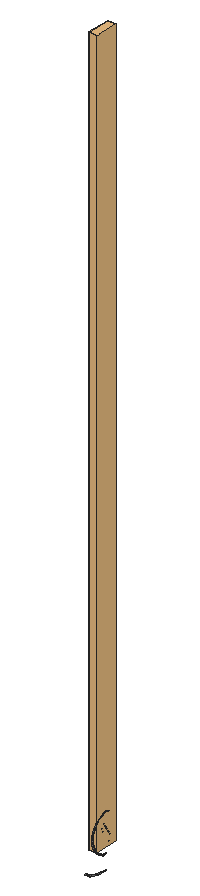
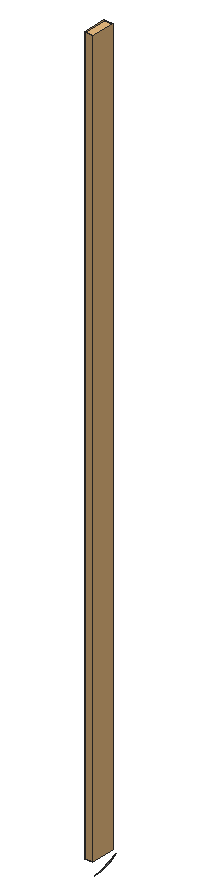
# SketchUp Ruby script. Lengths in inches.
U = 1.inch
M = Sketchup.active_model
def pt(a) = Geom::Point3d.new(a.map { |v| v * U })
def face(e, loops, mat)
  f = e.add_face(loops[0].map { |a| pt(a) })
  loops[1..].each { |l| e.add_face(l.map { |a| pt(a) }).erase! }
  f.material = f.back_material = mat if mat
  f
end
# faces: each face lists its corners as indices into pts; further lists are holes
def faces(e, pts, list, mat = nil) = list.each { |f| face(e, (f[0].is_a?(Array) ? f : [f]).map { |l| l.map { |i| pts[i] } }, mat) }
# xy, xz, yz: faces in a plane at the given z, y or x. An outline is a flat list of corners, or four numbers for a rectangle; further outlines are holes
def ring(l) = l.size == 4 ? [[l[0], l[1]], [l[2], l[1]], [l[2], l[3]], [l[0], l[3]]] : l.each_slice(2).to_a
def flat(e, list, mat, &to3) = list.each { |f| face(e, (f[0].is_a?(Array) ? f : [f]).map { |l| ring(l).map { |u, v| to3.(u, v) } }, mat) }
def xy(e, z, list, mat = nil) = flat(e, list, mat) { |x, y| [x, y, z] }
def xz(e, y, list, mat = nil) = flat(e, list, mat) { |x, z| [x, y, z] }
def yz(e, x, list, mat = nil) = flat(e, list, mat) { |y, z| [x, y, z] }
def lines(e, pts, list) = list.each { |a, b| e.add_line(pt(pts[a]), pt(pts[b])) }
# prism: a flat outline (further loops are holes) pulled along v
def prism(e, loops, v, mat = nil)
  f = face(e, loops, mat); d = Geom::Vector3d.new(v.map { |x| x * U })
  f.pushpull(f.normal.samedirection?(d) ? d.length : -d.length)
end
def box(e, o, s, mat = nil) = prism(e, [[o, [o[0] + s[0], o[1], o[2]], [o[0] + s[0], o[1] + s[1], o[2]], [o[0], o[1] + s[1], o[2]]]], [0, 0, s[2]], mat)
def at(x, y, z, deg = 0) = Geom::Transformation.translation(pt([x, y, z])) * Geom::Transformation.rotation(ORIGIN, Z_AXIS, deg.degrees)
def axes(o, x, y, z) = Geom::Transformation.new([*x, 0, *y, 0, *z, 0, *pt(o).to_a, 1])
def part(name) = M.definitions.add(name)
# library, detail: a bought-in or finely detailed component or shape, given as its bounding box
def library(name, o, s) = part(name).tap { |d| box(d.entities, o, s) }
def detail(e, o, s) = box(e.add_group.entities, o, s)
def put(e, d, t, mat = nil) = e.add_instance(d, t).tap { |i| i.material = mat if mat }
def group(e, t, mat = nil) = e.add_group.tap { |g| g.transformation = t; g.material = mat if mat }.entities
root = M.entities
M.materials.add("Material \#1").color = [140, 140, 140]
c1 = part("3DGeom~5_Defintion")
xy(c1.entities,-225.24,[[-0.79,-499.98,-2.33,-499.64,7.45,-496.14],[-0.79,-499.98,7.45,-496.14,1.58,-499.88],[1.58,-499.88,7.45,-496.14,3.84,-499.16],[-2.33,-499.64,7.4,-485.75,7.45,-496.14],[3.84,-499.16,7.45,-496.14,5.85,-497.89],
  [7.45,-496.14,7.4,-485.75,8.24,-487.08],[7.45,-496.14,8.24,-487.08,8.96,-489.34],[7.45,-496.14,8.96,-489.34,9.0625,-491.71],[7.45,-496.14,9.0625,-491.71,8.55,-494.03],[-7.4,-496.08,-8.24,-494.76,2.32,-482.2],
  [-8.24,-494.76,-8.96,-492.5,2.32,-482.2],[-8.96,-492.5,-9.0625,-490.125,2.32,-482.2],[-9.0625,-490.125,-8.55,-487.81,2.32,-482.2],[-8.55,-487.81,-7.45,-485.7,2.32,-482.2],[-7.45,-485.7,-5.85,-483.95,2.32,-482.2],
  [-5.85,-483.95,-3.84,-482.68,2.32,-482.2],[-3.84,-482.68,-1.58,-481.96,2.32,-482.2],[2.32,-482.2,-1.58,-481.96,0.79,-481.86],[0,481.82,-2.35,482.13,-6.92,496.71],[0,481.82,-6.92,496.71,1.55,482.04],
  [-2.35,482.13,-4.55,483.04,-6.92,496.71],[-4.55,483.04,-6.43,484.49,-6.92,496.71],[-6.43,484.49,-7.88,486.37,-6.92,496.71],[6.92,485.12,-1.55,499.8125,7.88,495.47],[6.92,485.12,7.88,495.47,7.88,486.37],
  [-7.88,486.37,-8.79,488.57,-6.92,496.71],[7.88,486.37,7.88,495.47,8.79,488.57],[-8.79,488.57,-9.1,490.92,-6.92,496.71],[8.79,488.57,7.88,495.47,9.1,490.92],[-9.1,490.92,-8.79,493.28,-6.92,496.71],
  [9.1,490.92,7.88,495.47,8.79,493.28],[-8.79,493.28,-7.88,495.47,-6.92,496.71],[7.88,495.47,-1.55,499.8125,0,500.02],[7.88,495.47,0,500.02,2.35,499.71],[7.88,495.47,2.35,499.71,4.55,498.8],
  [7.88,495.47,4.55,498.8,6.43,497.35]],"Material \#1")
xy(c1.entities,-221.57,[[-2.33,-499.64,-5.22,-498.37,7.4,-485.75],[-5.22,-498.37,-7.4,-496.08,5.22,-483.47],[-5.22,-498.37,5.22,-483.47,7.4,-485.75],[-7.4,-496.08,2.32,-482.2,5.22,-483.47],[1.55,482.04,-6.92,496.71,-4.55,498.8],
  [1.55,482.04,-4.55,498.8,4.55,483.04],[4.55,483.04,-4.55,498.8,-1.55,499.8125],[4.55,483.04,-1.55,499.8125,6.92,485.12]],"Material \#1")
xy(c1.entities,38.05,[[-2.33,-499.64,7.4,-485.75,-5.22,-498.37],[-5.22,-498.37,5.22,-483.47,-7.4,-496.08],[-5.22,-498.37,7.4,-485.75,5.22,-483.47],[-7.4,-496.08,5.22,-483.47,2.32,-482.2],[1.55,482.04,-4.55,498.8,-6.92,496.71],
  [1.55,482.04,4.55,483.04,-4.55,498.8],[4.55,483.04,-1.55,499.8125,-4.55,498.8],[4.55,483.04,6.92,485.12,-1.55,499.8125]],"Material \#1")
xy(c1.entities,41.72,[[-0.79,-499.98,7.45,-496.14,-2.33,-499.64],[-0.79,-499.98,1.58,-499.88,7.45,-496.14],[1.58,-499.88,3.84,-499.16,7.45,-496.14],[-2.33,-499.64,7.45,-496.14,7.4,-485.75],[3.84,-499.16,5.85,-497.89,7.45,-496.14],
  [7.45,-496.14,8.24,-487.08,7.4,-485.75],[7.45,-496.14,8.55,-494.03,9.0625,-491.71],[7.45,-496.14,8.96,-489.34,8.24,-487.08],[7.45,-496.14,9.0625,-491.71,8.96,-489.34],[-7.4,-496.08,2.32,-482.2,-8.24,-494.76],
  [-8.24,-494.76,2.32,-482.2,-8.96,-492.5],[-8.96,-492.5,2.32,-482.2,-9.0625,-490.125],[-9.0625,-490.125,2.32,-482.2,-8.55,-487.81],[-8.55,-487.81,2.32,-482.2,-7.45,-485.7],[-7.45,-485.7,2.32,-482.2,-5.85,-483.95],
  [-5.85,-483.95,2.32,-482.2,-3.84,-482.68],[-3.84,-482.68,2.32,-482.2,-1.58,-481.96],[2.32,-482.2,0.79,-481.86,-1.58,-481.96],[0,481.82,-6.92,496.71,-2.35,482.13],[0,481.82,1.55,482.04,-6.92,496.71],
  [-2.35,482.13,-6.92,496.71,-4.55,483.04],[-4.55,483.04,-6.92,496.71,-6.43,484.49],[-6.43,484.49,-6.92,496.71,-7.88,486.37],[6.92,485.12,7.88,495.47,-1.55,499.8125],[6.92,485.12,7.88,486.37,7.88,495.47],
  [-7.88,486.37,-6.92,496.71,-8.79,488.57],[7.88,486.37,8.79,488.57,7.88,495.47],[-8.79,488.57,-6.92,496.71,-9.1,490.92],[8.79,488.57,9.1,490.92,7.88,495.47],[-9.1,490.92,-6.92,496.71,-8.79,493.28],
  [9.1,490.92,8.79,493.28,7.88,495.47],[-8.79,493.28,-6.92,496.71,-7.88,495.47],[7.88,495.47,0,500.02,-1.55,499.8125],[7.88,495.47,2.35,499.71,0,500.02],[7.88,495.47,4.55,498.8,2.35,499.71],
  [7.88,495.47,6.43,497.35,4.55,498.8]],"Material \#1")
c2 = library("3DGeom~4_Defintion",[-18.02,-499.97,-221.16],[36.04,1000,262.12])
yz(root,362.685,[[201.798,43.518,201.655,43.532,201.658,43.547],[201.798,43.518,201.658,43.547,201.798,43.533],[201.655,43.532,201.522,43.572,201.526,43.586],[201.655,43.532,201.526,43.586,201.658,43.547],[201.522,43.572,201.399,43.636,201.405,43.649],
  [201.522,43.572,201.405,43.649,201.526,43.586],[201.798,43.749,201.751,43.754,201.753,43.768],[201.798,43.749,201.753,43.768,201.798,43.764],[201.751,43.754,201.706,43.767,201.711,43.781],[201.751,43.754,201.711,43.781,201.753,43.768],
  [201.706,43.767,201.665,43.788,201.672,43.801],[201.706,43.767,201.672,43.801,201.711,43.781],[201.665,43.788,201.628,43.817,201.637,43.828],[201.665,43.788,201.637,43.828,201.672,43.801],[201.628,43.817,201.597,43.851,201.607,43.861],
  [201.628,43.817,201.607,43.861,201.637,43.828],[201.597,43.851,201.571,43.891,201.583,43.898],[201.597,43.851,201.583,43.898,201.607,43.861],[201.571,43.891,201.551,43.936,201.564,43.941],[201.571,43.891,201.564,43.941,201.583,43.898],
  [201.551,43.936,201.539,43.984,201.552,43.987],[201.551,43.936,201.552,43.987,201.564,43.941],[201.539,43.984,201.535,44.036,201.548,44.036],[201.539,43.984,201.548,44.036,201.552,43.987],[201.535,44.036,201.539,44.087,201.552,44.084],
  [201.535,44.036,201.552,44.084,201.548,44.036],[201.552,44.084,201.539,44.087,201.564,44.13],[201.539,44.087,201.551,44.135,201.564,44.13],[201.564,44.13,201.551,44.135,201.583,44.173],[201.551,44.135,201.571,44.18,201.583,44.173],
  [201.583,44.173,201.571,44.18,201.607,44.211],[201.571,44.18,201.597,44.22,201.607,44.211],[201.607,44.211,201.597,44.22,201.637,44.243],[201.597,44.22,201.628,44.255,201.637,44.243],[201.637,44.243,201.628,44.255,201.672,44.27],
  [201.628,44.255,201.665,44.283,201.672,44.27],[201.672,44.27,201.665,44.283,201.711,44.29],[201.665,44.283,201.706,44.304,201.711,44.29],[201.711,44.29,201.706,44.304,201.753,44.303],[201.753,44.303,201.706,44.304,201.751,44.318],
  [201.753,44.303,201.751,44.318,201.798,44.307],[201.842,44.303,201.798,44.307,201.798,44.322],[201.798,44.307,201.751,44.318,201.798,44.322]],"Material \#1")
p = [[362.566,201.821,43.942],[362.567,201.821,43.942],[362.567,201.725,44.091],[362.566,201.725,44.091],[362.685,201.821,43.942],[362.685,201.725,44.091],
  [362.684,201.725,44.091],[362.684,201.821,43.942],[362.566,201.858,43.883],[362.568,201.858,43.883],[362.568,201.838,43.914],[362.566,201.838,43.914],
  [362.685,201.858,43.883],[362.685,201.838,43.914],[362.684,201.838,43.914],[362.683,201.858,43.883],[362.566,201.889,43.953],[362.568,201.889,43.953],
  [362.568,201.908,43.922],[362.566,201.908,43.922],[362.568,201.886,43.899],[362.566,201.886,43.899],[362.685,201.889,43.953],[362.685,201.908,43.922],
  [362.683,201.908,43.922],[362.684,201.889,43.953],[362.685,201.886,43.899],[362.683,201.886,43.899],[362.566,201.775,44.129],[362.567,201.775,44.129],
  [362.567,201.871,43.98],[362.566,201.871,43.98],[362.685,201.775,44.129],[362.685,201.871,43.98],[362.684,201.871,43.98],[362.684,201.775,44.129],
  [362.568,201.707,44.119],[362.566,201.707,44.119],[362.568,201.687,44.149],[362.566,201.687,44.149],[362.568,201.71,44.172],[362.566,201.71,44.172],
  [362.685,201.707,44.119],[362.684,201.707,44.119],[362.685,201.687,44.149],[362.683,201.687,44.149],[362.685,201.71,44.172],[362.683,201.71,44.172],
  [362.566,201.757,44.157],[362.568,201.757,44.157],[362.685,201.757,44.157],[362.684,201.757,44.157],[362.568,201.737,44.188],[362.566,201.737,44.188],
  [362.685,201.737,44.188],[362.683,201.737,44.188]]
faces(root,p,[[0,1,2],[2,3,0],[4,5,6],[6,7,4],[8,9,10],[10,11,8],[11,10,1],[1,0,11],
  [12,13,14],[14,15,12],[13,4,7],[7,14,13],[16,17,18],[18,19,16],[19,18,20],[20,21,19],
  [21,20,9],[9,8,21],[22,23,24],[24,25,22],[23,26,27],[27,24,23],[26,12,15],[15,27,26],
  [28,29,30],[30,31,28],[32,33,34],[34,35,32],[31,30,17],[17,16,31],[33,22,25],[25,34,33],
  [3,2,36],[36,37,3],[37,36,38],[38,39,37],[39,38,40],[40,41,39],[5,42,43],[43,6,5],
  [42,44,45],[45,43,42],[44,46,47],[47,45,44],[48,49,29],[29,28,48],[50,32,35],[35,51,50],
  [41,40,52],[52,53,41],[53,52,49],[49,48,53],[46,54,55],[55,47,46],[54,50,51],[51,55,54]],"Material \#1")
put(root,c1,axes([362.67,201.8,49.3125],[0,-0.00986,0],[0,0,0.01075],[0.00045,0,0]),"Material \#1")
put(root,c2,axes([362.67,201.8,49.3125],[0,-0.01004,0],[0,0,0.01095],[0.00046,0,0]),"Material \#1")
